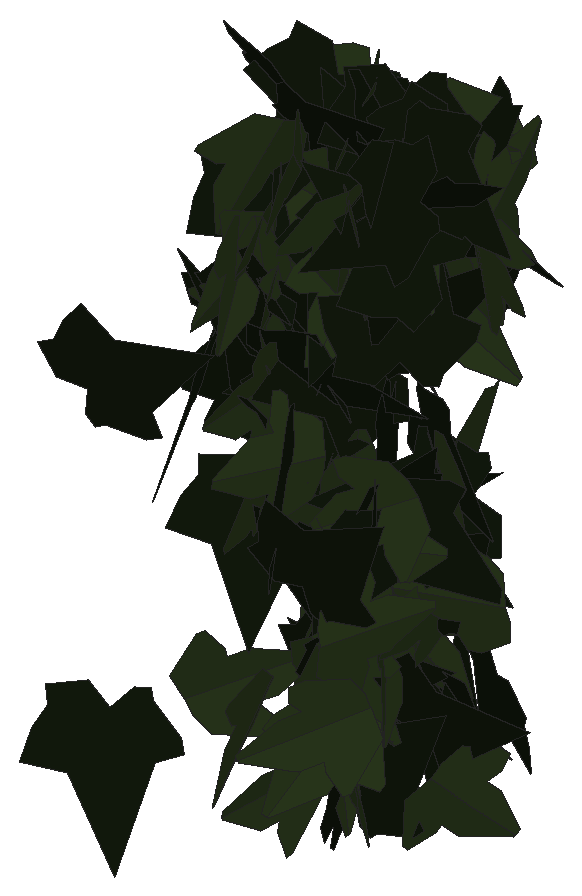
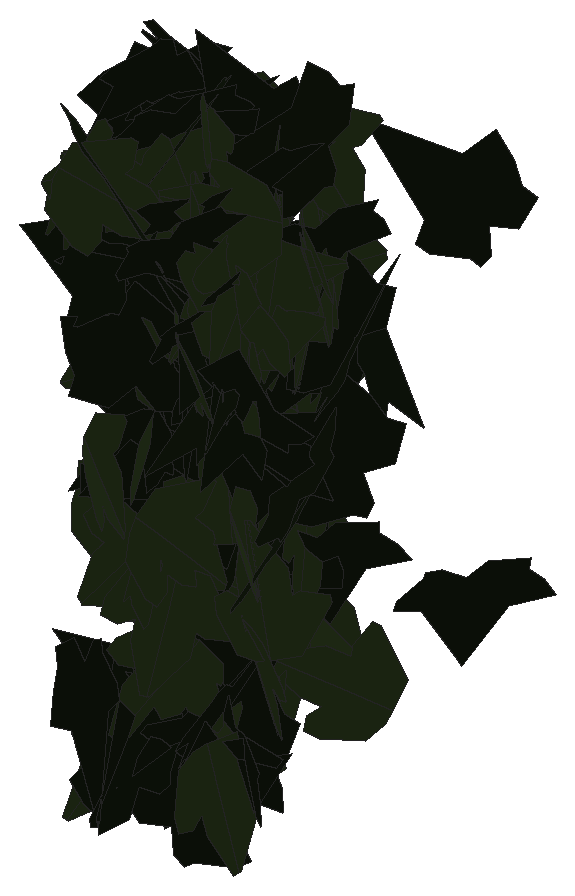
# SketchUp Ruby script. Lengths in inches.
U = 1.inch
M = Sketchup.active_model
def pt(a) = Geom::Point3d.new(a.map { |v| v * U })
def face(e, loops, mat)
  f = e.add_face(loops[0].map { |a| pt(a) })
  loops[1..].each { |l| e.add_face(l.map { |a| pt(a) }).erase! }
  f.material = f.back_material = mat if mat
  f
end
# faces: each face lists its corners as indices into pts; further lists are holes
def faces(e, pts, list, mat = nil) = list.each { |f| face(e, (f[0].is_a?(Array) ? f : [f]).map { |l| l.map { |i| pts[i] } }, mat) }
# xy, xz, yz: faces in a plane at the given z, y or x. An outline is a flat list of corners, or four numbers for a rectangle; further outlines are holes
def ring(l) = l.size == 4 ? [[l[0], l[1]], [l[2], l[1]], [l[2], l[3]], [l[0], l[3]]] : l.each_slice(2).to_a
def flat(e, list, mat, &to3) = list.each { |f| face(e, (f[0].is_a?(Array) ? f : [f]).map { |l| ring(l).map { |u, v| to3.(u, v) } }, mat) }
def xy(e, z, list, mat = nil) = flat(e, list, mat) { |x, y| [x, y, z] }
def xz(e, y, list, mat = nil) = flat(e, list, mat) { |x, z| [x, y, z] }
def yz(e, x, list, mat = nil) = flat(e, list, mat) { |y, z| [x, y, z] }
def lines(e, pts, list) = list.each { |a, b| e.add_line(pt(pts[a]), pt(pts[b])) }
# prism: a flat outline (further loops are holes) pulled along v
def prism(e, loops, v, mat = nil)
  f = face(e, loops, mat); d = Geom::Vector3d.new(v.map { |x| x * U })
  f.pushpull(f.normal.samedirection?(d) ? d.length : -d.length)
end
def box(e, o, s, mat = nil) = prism(e, [[o, [o[0] + s[0], o[1], o[2]], [o[0] + s[0], o[1] + s[1], o[2]], [o[0], o[1] + s[1], o[2]]]], [0, 0, s[2]], mat)
def at(x, y, z, deg = 0) = Geom::Transformation.translation(pt([x, y, z])) * Geom::Transformation.rotation(ORIGIN, Z_AXIS, deg.degrees)
def axes(o, x, y, z) = Geom::Transformation.new([*x, 0, *y, 0, *z, 0, *pt(o).to_a, 1])
def part(name) = M.definitions.add(name)
# library, detail: a bought-in or finely detailed component or shape, given as its bounding box
def library(name, o, s) = part(name).tap { |d| box(d.entities, o, s) }
def detail(e, o, s) = box(e.add_group.entities, o, s)
def put(e, d, t, mat = nil) = e.add_instance(d, t).tap { |i| i.material = mat if mat }
def group(e, t, mat = nil) = e.add_group.tap { |g| g.transformation = t; g.material = mat if mat }.entities
root = M.entities
M.materials.add("efeu1").color = [18, 25, 13]
M.materials.add("efeu2").color = [43, 57, 29]
c1 = part("ivyleaf_9")
p = [[1.54,2.16,1.25],[1.36,2.04,1.19],[-0.21,0.99,0.68],[-0.71,1.11,0.82],[-0.85,0.86,0.67],[-0.8,0.17,0.21],
  [-0.9,-0.01,0.1],[-0.67,-0.16,-0.02],[-0.08,-0.08,-0.05],[-0.03,-0.6,-0.4],[0.65,-0.88,-0.66],[0.83,-0.6,-0.49],
  [1.29,-0.42,-0.43],[1.8125,-0.07,-0.26],[1.21,0.44,0.15]]
faces(c1.entities,p,[[0,1,2,3,4,5,6,7,8,9,10,11,12,13,14]],"efeu1")
c2 = part("ivyleaf_10")
p = [[0,0.5,-0.03],[-0.0625,2.02,-0.43],[-0.19,2.01,-0.46],[-0.54,1.05,-0.29],[-0.52,0.625,-0.18],[-0.83,0.76,-0.28],
  [-1.16,0.64,-0.33],[-1.15,0.33,-0.24],[-0.77,-0.39,0.02],[-0.3,-0.51,0.16],[0.04,-0.48,0.23],[-0.02,2.01,-0.4375],
  [-0.06,2.01,-0.43],[0.04,-0.49,0.23],[0.67,-0.49,0.14],[1.38,0.36,-0.2],[1.375,0.51,-0.24],[0.81,0.65,-0.19],
  [0.62,0.59,-0.15],[0.6,1.09,-0.28],[0.5,1.23,-0.31]]
faces(c2.entities,p,[[0,1,2,3,4,5,6,7,8,9,10],[11,12,0,13,14,15,16,17,18,19,20]],"efeu2")
put(root,c1,axes([26.17,222.62,210.74],[0.16285,0.0009,0.47274],[0.47272,-0.00413,-0.16283],[0.00361,0.49998,-0.00219]))
put(root,c1,axes([26.61,221.9,211.7],[-0.299,0.15439,-0.36982],[0.31819,-0.18905,-0.33618],[-0.24363,-0.43638,0.0148]))
put(root,c1,axes([26.43,223.62,210.13],[0.05085,-0.39738,0.29918],[0.0403,-0.29645,-0.40061],[0.49577,0.06486,0.00187]))
put(root,c1,axes([26.73,222.37,211.34],[0.13991,-0.44603,0.17743],[-0.03757,0.17407,0.46721],[-0.47855,-0.14407,0.01519]))
put(root,c1,axes([26.56,222.69,209.89],[-0.24498,-0.39685,-0.18025],[0.10032,0.14988,-0.46634],[0.42417,-0.26465,0.00619]))
put(root,c1,axes([26.82,223.59,211.56],[-0.49386,0.06546,0.04259],[0.04104,-0.01442,0.4981],[0.06644,0.49549,0.00887]))
put(root,c1,axes([26.37,223.23,210.66],[0.11385,-0.33946,0.34901],[0.15332,-0.31519,-0.35658],[0.46209,0.18821,0.03232]))
put(root,c1,axes([26.55,220.52,208.52],[-0.17039,-0.42889,-0.19241],[0.07799,0.17603,-0.46144],[0.46356,-0.18727,0.00691]))
put(root,c2,axes([26.7,223.56,212.33],[-0.34285,-0.35172,-0.09353],[-0.05672,-0.07529,0.49103],[-0.3595,0.34731,0.01173]))
put(root,c2,axes([26.58,223.41,209.25],[-0.46251,-0.0941,0.16501],[0.168,0.00007,0.47093],[-0.08865,0.49107,0.03155]))
put(root,c2,axes([26.71,222.61,210.05],[0.03257,-0.4567,-0.20091],[0.0211,0.20242,-0.45671],[0.49849,0.02127,0.03246]))
put(root,c2,axes([26.47,222.11,208.01],[-0.14514,-0.17857,0.4439],[0.28518,0.34019,0.2301],[-0.3842,0.31997,0.0031]))
put(root,c1,axes([26.57,222.73,213.15],[-0.04749,-0.45954,-0.19123],[0.02534,0.18962,-0.46195],[0.49709,-0.05357,0.00528]))
put(root,c2,axes([26.81,223.9,207.91],[-0.12899,-0.47806,0.06942],[-0.02076,-0.0663,-0.49515],[0.48263,-0.13062,-0.00275]))
put(root,c2,axes([26.77,222.54,212.93],[0.19917,-0.45327,-0.06984],[-0.02871,0.06367,-0.4951],[0.45772,0.20122,-0.00066]))
put(root,c1,axes([26.37,222.87,214.1875],[0.37975,-0.23814,0.22154],[0.19105,-0.1123,-0.44821],[0.26323,0.42506,0.00571]))
put(root,c2,axes([26.72,223.39,213.05],[-0.28934,-0.35489,-0.20083],[0.13306,0.15061,-0.45784],[0.38546,-0.31839,0.00728]))
put(root,c2,axes([26.47,223.7,212.75],[0.3605,-0.05675,0.34178],[0.33953,-0.04033,-0.36482],[0.06897,0.49513,0.00946]))
put(root,c2,axes([26.99,222.3,211.92],[-0.01817,0.07692,0.49371],[-0.34311,0.35723,-0.06829],[-0.36324,-0.34128,0.03981]))
put(root,c2,axes([26.71,222.37,212.51],[0.01609,-0.11059,0.48735],[0.15839,-0.46134,-0.10992],[0.47398,0.15792,0.02019]))
put(root,c2,axes([26.77,223.36,209.04],[0.3873,-0.31618,0.00527],[0.00407,-0.00335,-0.49997],[0.31619,0.38733,-0.00003]))
put(root,c2,axes([26.58,222.82,213.16],[0.31779,-0.21999,0.3172],[0.26792,-0.1701,-0.38638],[0.27791,0.41554,0.00977]))
put(root,c2,axes([26.75,222.3,212.65],[0.02679,0.39052,-0.31109],[-0.0218,-0.31032,-0.39144],[-0.49881,0.03453,0.0004]))
put(root,c2,axes([27.07,223.27,212.69],[0.06772,0.08301,0.48839],[-0.30092,-0.38468,0.10711],[0.39353,-0.30844,-0.00215]))
put(root,c2,axes([26.91,222.375,213.78],[-0.12122,-0.43224,0.22017],[-0.05198,-0.21406,-0.44886],[0.48229,-0.13171,0.00696]))
put(root,c1,axes([27,223.26,211.625],[-0.12961,0.1107,-0.47005],[-0.35378,0.3095,0.17044],[0.3287,0.37677,-0.0019]))
put(root,c2,axes([26.88,222.42,212.07],[-0.41925,-0.26433,-0.06601],[-0.05587,-0.03515,0.49562],[-0.26666,0.42296,-0.00006]))
put(root,c1,axes([26.8,223.47,213.89],[-0.17872,-0.44691,0.13538],[-0.03161,-0.13304,-0.48094],[0.4659,-0.18047,0.0193]))
put(root,c1,axes([26.54,222.29,211.88],[0.17796,0.00183,0.46725],[0.46715,-0.01124,-0.17788],[0.00985,0.49987,-0.00571]))
put(root,c2,axes([26.89,223.4,210.18],[0.28334,-0.3892,0.13506],[0.07949,-0.1092,-0.48141],[0.40423,0.29428,-0.00001]))
put(root,c2,axes([26.61,223.58,213.65],[-0.05552,0.0027,-0.4969],[0.49367,-0.0567,-0.05547],[-0.05664,-0.49677,0.00362]))
put(root,c1,axes([26.75,223.78,211.89],[0.39734,-0.29675,-0.06375],[-0.04947,0.04031,-0.49591],[0.29946,0.40039,0.00268]))
put(root,c1,axes([26.71,222.87,212.0625],[0.30173,-0.39293,0.06761],[0.03483,-0.05849,-0.49534],[0.39718,0.30363,-0.00793]))
put(root,c2,axes([26.64,223.625,211.84],[-0.02809,0.00711,0.49916],[0.48941,-0.09821,0.02894],[0.09845,0.49021,-0.00144]))
put(root,c2,axes([26.98,222.85,212.16],[0.05224,-0.37634,0.32503],[0.10389,-0.31134,-0.37719],[0.48629,0.10695,0.04567]))
put(root,c1,axes([27.3125,223.84,207.17],[0.08373,-0.03379,0.49178],[-0.47208,0.13808,0.08987],[-0.14188,-0.47937,-0.00878]))
put(root,c1,axes([26.65,220.16,212.11],[0.03007,-0.01545,0.49886],[0.46411,-0.18295,-0.03365],[0.18357,0.46507,0.00334]))
put(root,c2,axes([27.14,222.42,213.66],[0.08173,-0.32712,-0.36921],[-0.0799,0.36052,-0.33711],[0.48676,0.1141,0.00666]))
put(root,c1,axes([27.08,222.48,209.71],[0.3855,0.18856,-0.25659],[-0.23497,-0.10345,-0.42905],[-0.21489,0.45138,0.00885]))
put(root,c1,axes([26.94,223.17,211.03],[-0.31527,-0.22643,-0.31517],[0.25376,0.18695,-0.38815],[0.29362,-0.4047,-0.00296]))
put(root,c1,axes([26.85,223.56,208.18],[-0.20134,-0.00646,-0.45763],[0.45766,0.00086,-0.20136],[0.00339,-0.49996,0.00556]))
put(root,c2,axes([27.08,222.23,211.36],[-0.03021,0.00692,-0.49904],[-0.09554,-0.49079,-0.00102],[-0.48986,0.09529,0.03097]))
put(root,c1,axes([26.91,223.55,208.57],[0.21902,-0.39966,-0.20567],[-0.10038,0.17952,-0.45574],[0.43813,0.24092,-0.0016]))
put(root,c1,axes([26.91,223.73,208.07],[-0.18921,-0.24159,-0.39476],[0.28116,0.27875,-0.30536],[0.36762,-0.33754,0.03036]))
put(root,c1,axes([27.39,222.8125,211.81],[-0.19338,0.14226,-0.4386],[-0.37892,0.22197,0.23906],[0.26273,0.42484,0.02196]))
put(root,c1,axes([27.05,223.83,212.6],[-0.08661,-0.47526,0.12893],[-0.01805,-0.12776,-0.48307],[0.49211,-0.08833,0.00497]))
put(root,c2,axes([27.08,223.61,212.87],[0.17,-0.46295,-0.08236],[0.02854,-0.07725,0.49317],[-0.46935,-0.17238,0.00016]))
put(root,c1,axes([27.18,224.05,213.43],[-0.20975,-0.45383,0.00682],[0.00304,-0.00892,-0.49991],[0.45387,-0.20967,0.0065]))
put(root,c2,axes([27.12,223.93,212.1875],[0.36105,-0.30275,0.16728],[0.13199,-0.10293,-0.47115],[0.31972,0.38438,0.00559]))
put(root,c1,axes([26.84,223.33,207.8],[0.12129,-0.04112,0.48332],[0.44543,-0.1878,-0.12776],[0.19205,0.46156,-0.00892]))
put(root,c2,axes([26.99,223.54,211.42],[-0.15248,0.09097,0.46741],[0.40194,-0.23857,0.17756],[0.25533,0.42989,-0.00037]))
put(root,c1,axes([27.39,223.19,212.24],[0.00918,0.37993,0.32491],[-0.00873,0.32504,-0.37983],[-0.49984,0.0013,0.0126]))
put(root,c2,axes([27.26,223.11,212.69],[-0.05645,0.32084,0.37931],[-0.05751,0.37497,-0.32572],[-0.49346,-0.0804,-0.00543]))
put(root,c2,axes([27.38,222.23,210.68],[-0.07152,0.10628,0.48331],[0.0082,-0.48801,0.10853],[0.49479,0.02345,0.06806]))
put(root,c2,axes([27.32,221.69,208.41],[0.16962,-0.34433,0.32041],[0.12132,-0.29705,-0.38346],[0.45443,0.20783,-0.01722]))
put(root,c2,axes([27.17,223.5,207.66],[-0.25968,0.05327,0.42394],[0.36467,-0.23091,0.25239],[0.22268,0.44027,0.08107]))
put(root,c2,axes([27.5,223.08,214.14],[0.15363,-0.4324,-0.19857],[-0.06775,0.18666,-0.45888],[0.47097,0.1679,-0.00124]))
put(root,c1,axes([27.59,223.03,211.4],[-0.04342,-0.28725,-0.40694],[-0.00307,-0.40833,0.28855],[-0.4981,0.02756,0.0337]))
put(root,c2,axes([27.04,222.81,213.04],[0.06665,0.02183,0.49506],[0.47473,0.1404,-0.0701],[-0.14208,0.47939,-0.00201]))
put(root,c1,axes([27.13,222.74,213.76],[0.44945,0.0194,-0.21822],[0.21512,0.05529,0.44796],[0.04151,-0.49656,0.04135]))
put(root,c1,axes([27.32,222.09,210.96],[-0.17708,-0.00608,-0.46755],[0.4513,-0.13304,-0.16919],[-0.12235,-0.48194,0.05261]))
put(root,c1,axes([27.09,222.31,211.55],[0.36588,-0.0643,0.33466],[0.33245,-0.04054,-0.37126],[0.07488,0.49419,0.01309]))
put(root,c1,axes([27.22,223.35,213.31],[0.07971,-0.25879,-0.42032],[0.16006,0.41631,-0.22597],[0.46693,-0.09853,0.14921]))
put(root,c2,axes([27.5,222.84,209.9],[-0.29594,-0.40274,-0.01499],[-0.00129,-0.01765,0.49969],[-0.40301,0.29579,0.00941]))
put(root,c1,axes([27.46,223.01,212.57],[-0.1235,-0.46146,0.14767],[-0.02387,-0.14641,-0.47749],[0.48392,-0.12499,0.01413]))
put(root,c2,axes([27.49,222.67,207.79],[-0.02474,0.49661,-0.05256],[-0.00154,-0.0527,-0.49721],[-0.49939,-0.02444,0.00414]))
put(root,c1,axes([27.62,222.47,206.99],[0.0529,-0.09327,0.48837],[0.1044,0.48226,0.08079],[-0.48611,0.09343,0.0705]))
put(root,c1,axes([27.6,222.71,208.75],[0.22704,0.44385,0.03807],[0.01667,0.03423,-0.49855],[-0.44517,0.22765,0.00075]))
put(root,c2,axes([27.73,223.6,209.96],[-0.02025,-0.35618,0.35032],[-0.02928,-0.34916,-0.3567],[0.49873,-0.03497,-0.00672]))
put(root,c2,axes([27.51,222.54,208.58],[-0.42571,-0.00681,-0.26215],[0.26207,0.00693,-0.42576],[0.00943,-0.49991,-0.00233]))
put(root,c1,axes([28.08,223.63,212.52],[-0.34273,0.1301,0.34002],[-0.32111,0.11202,-0.36653],[-0.17154,-0.4696,0.00677]))
put(root,c2,axes([27.73,223.41,209.25],[-0.46418,-0.17554,-0.06101],[0.05644,0.02321,-0.49626],[0.17706,-0.4676,-0.00173]))
put(root,c2,axes([27.76,221.8,207.72],[-0.00342,0.01262,-0.49983],[-0.15199,-0.47621,-0.01099],[-0.47633,0.15186,0.0071]))
put(root,c2,axes([27.59,223.45,208.6],[-0.41899,-0.08519,-0.25921],[0.25243,0.05927,-0.42751],[0.10357,-0.48911,-0.00666]))
put(root,c1,axes([27.74,223.89,211.7],[0.34593,0.11689,0.34157],[-0.32158,-0.11523,0.36511],[0.16408,-0.47229,-0.00454]))
put(root,c2,axes([27.52,223.26,212.31],[-0.27243,0.0022,0.41926],[0.41918,0.01135,0.27232],[-0.00832,0.49987,-0.00803]))
put(root,c2,axes([27.89,222.47,212.73],[0.38533,0.25472,-0.1914],[-0.16178,-0.10234,-0.4619],[-0.27449,0.4179,0.00354]))
put(root,c1,axes([28.17,222.58,213.44],[-0.47342,-0.12768,-0.09784],[-0.09464,-0.0248,0.49033],[-0.13006,0.48279,-0.00069]))
put(root,c2,axes([27.89,222.41,207.24],[-0.41132,0.25837,0.11859],[0.09753,-0.06767,0.4857],[0.26703,0.42269,0.00527]))
put(root,c1,axes([27.62,222.79,207.1],[-0.14312,0.06557,0.47457],[0.39325,-0.26681,0.15546],[0.27363,0.41775,0.02481]))
put(root,c1,axes([27.64,223.25,214.06],[0.22911,-0.44398,0.01987],[0.01278,-0.01577,-0.49959],[0.44424,0.22942,0.00412]))
put(root,c1,axes([27.5625,222.64,209.47],[0.31401,-0.12379,-0.36888],[0.35745,-0.09548,0.33632],[-0.15371,-0.47493,0.02853]))
put(root,c2,axes([27.875,223.23,213.68],[0.28411,0.39303,-0.12171],[-0.08054,-0.09192,-0.48483],[-0.40348,0.29509,0.01108]))
put(root,c1,axes([27.8,223.23,214.15],[-0.11782,-0.46469,-0.14205],[0.03113,0.13865,-0.47938],[0.48492,-0.1218,-0.00374]))
put(root,c1,axes([27.64,224,207.56],[0.46096,-0.1147,-0.15607],[0.1563,-0.01764,0.47461],[-0.11438,-0.48635,0.01959]))
put(root,c2,axes([28.3,223.99,213.59],[-0.16842,-0.11853,0.45562],[-0.34684,-0.29596,-0.20521],[0.31834,-0.38517,0.01747]))
put(root,c2,axes([27.87,222.95,208.73],[-0.09098,0.37961,-0.31245],[0.08435,-0.30099,-0.39025],[-0.48436,-0.12371,-0.00927]))
put(root,c2,axes([28.06,222.02,213.625],[-0.11435,-0.48505,-0.04058],[0.00527,0.04045,-0.49833],[0.48672,-0.11439,-0.00414]))
put(root,c1,axes([28.14,223.57,207.14],[-0.06621,-0.28754,0.40365],[0.13509,0.38135,0.29381],[-0.47683,0.14796,0.02718]))
put(root,c2,axes([27.95,222.23,213.52],[-0.2488,0.37033,-0.22573],[0.11555,-0.19423,-0.44601],[-0.41803,-0.2741,0.01106]))
put(root,c2,axes([27.75,223.59,213.34],[-0.16853,-0.08475,0.46305],[0.42561,0.18272,0.18834],[-0.20114,0.45764,0.01055]))
put(root,c1,axes([27.9,222.89,211.125],[-0.08364,0.0526,-0.49014],[0.43778,-0.22061,-0.09838],[-0.22661,-0.4456,-0.00915]))
put(root,c2,axes([27.81,223.64,211.81],[0.21812,0.11261,0.4356],[0.39599,0.18175,-0.24527],[-0.21358,0.45198,-0.0099]))
put(root,c2,axes([28.48,222.22,210.625],[0.27616,-0.00071,-0.41682],[-0.41165,0.07799,-0.27287],[0.0654,0.49388,0.04249]))
put(root,c1,axes([28.54,223.48,213.63],[-0.27868,0.3462,0.22908],[-0.13841,0.18264,-0.44439],[-0.39138,-0.3111,-0.00596]))
put(root,c2,axes([28.17,223.9375,210.74],[0.19972,-0.42067,0.18207],[0.09667,-0.15547,-0.46528],[0.44807,0.22105,0.01923]))
put(root,c2,axes([28.05,223.54,209.66],[-0.37779,0.16182,-0.28477],[0.26304,-0.10914,-0.41098],[-0.19517,-0.46033,-0.00266]))
put(root,c1,axes([28.56,223.17,210.3125],[-0.13626,-0.21746,-0.42912],[-0.19751,-0.38139,0.25599],[-0.43866,0.23927,0.01804]))
put(root,c2,axes([28.48,221.51,208.7],[0.12869,0.11251,-0.46987],[-0.37614,-0.28187,-0.17051],[-0.30325,0.39736,0.01209]))
put(root,c1,axes([28.12,222.4375,210.26],[0.18933,0.23912,0.3962],[0.23952,0.31564,-0.30496],[-0.39596,0.30527,0.00498]))
put(root,c2,axes([28.35,221.54,208.57],[0.304,0.26365,-0.29676],[-0.22117,-0.19791,-0.40239],[-0.32965,0.37592,-0.00371]))
put(root,c1,axes([28.26,223.26,213.84],[-0.21369,-0.42935,0.1414],[-0.05618,-0.12997,-0.47953],[0.44853,-0.22083,0.0073]))
put(root,c2,axes([28.25,223.2,209.16],[-0.00413,-0.04106,0.49829],[0.16037,-0.47209,-0.03757],[0.47356,0.15952,0.01707]))
put(root,c1,axes([27.94,223.15,207.75],[0.1279,-0.05738,0.47995],[0.42079,-0.23108,-0.13976],[0.23786,0.43967,-0.01082]))
put(root,c1,axes([27.95,223.875,212.79],[0.25917,-0.25474,0.34343],[0.29152,-0.18852,-0.35983],[0.31281,0.38674,0.05081]))
put(root,c1,axes([28.0625,221.47,209.99],[-0.11324,-0.06043,0.48325],[0.41409,-0.27308,0.06289],[0.25633,0.41446,0.11189]))
put(root,c2,axes([28.25,222.36,213.375],[0.12269,0.42821,0.22712],[0.06557,0.21747,-0.44543],[-0.48026,0.13908,-0.00279]))
put(root,c2,axes([28,222.33,210.01],[0.0892,-0.0706,-0.48689],[0.47788,-0.10516,0.1028],[-0.11692,-0.48369,0.04872]))
put(root,c1,axes([28.57,223.61,208.24],[0.23204,0.02557,-0.44216],[-0.4413,-0.02893,-0.23327],[-0.03751,0.49851,0.00914]))
put(root,c2,axes([28.27,221.72,209.4],[0.0017,-0.02643,-0.4993],[0.24581,0.43484,-0.02218],[0.4354,-0.24539,0.01447]))
put(root,c1,axes([28.44,222.37,212.09],[-0.38914,-0.10648,0.29535],[0.28576,0.07469,0.40344],[-0.13003,0.48279,0.00273]))
put(root,c1,axes([28.16,223.09,209.21],[-0.14507,-0.03097,0.47749],[0.37198,-0.32114,0.09218],[0.30097,0.38198,0.11622]))
put(root,c2,axes([28.43,223.34,212.9],[-0.48115,-0.11119,-0.07828],[0.07591,0.01919,-0.49383],[0.11283,-0.4871,-0.00159]))
put(root,c1,axes([28.3125,222.54,212.14],[0.07572,0.10053,0.4839],[0.33876,0.34591,-0.12487],[-0.35988,0.34676,-0.01573]))
put(root,c1,axes([28.77,222.34,213.18],[-0.29235,-0.38635,-0.12355],[-0.07372,-0.09915,0.48449],[-0.39887,0.3015,0.00101]))
put(root,c1,axes([28.12,223.14,210.91],[0.08292,-0.05119,-0.49041],[0.49116,0.05236,0.07759],[0.04341,-0.49461,0.05896]))
put(root,c2,axes([28.34,223.1,210.66],[-0.29011,0.30654,-0.26809],[0.17814,-0.20047,-0.42199],[-0.36621,-0.34036,0.00711]))
put(root,c2,axes([28.66,223.31,212.81],[-0.44178,0.19036,0.13635],[-0.12656,0.05084,-0.48104],[-0.19701,-0.45954,0.00327]))
put(root,c2,axes([28.48,222.99,207.36],[-0.2077,-0.30243,-0.3397],[0.2007,0.27418,-0.3668],[0.40814,-0.28873,0.0075]))
put(root,c1,axes([28.5625,222.3,213.66],[0.26143,0.42218,0.0585],[0.03126,0.04945,-0.49657],[-0.42506,0.26329,-0.00054]))
put(root,c1,axes([28.89,222.02,213.97],[-0.47488,0.13158,0.08472],[-0.08029,0.02749,-0.49274],[-0.13432,-0.48159,-0.00498]))
put(root,c1,axes([28.35,222.27,210.44],[0.00554,-0.09489,-0.49088],[0.17233,0.46119,-0.08721],[0.46933,-0.16822,0.03781]))
put(root,c1,axes([28.44,222.48,214.18],[0.1294,-0.28194,-0.39213],[-0.02199,0.4021,-0.29637],[0.48246,0.09394,0.09166]))
put(root,c2,axes([29.02,222.88,209.51],[-0.06891,-0.00994,0.49513],[-0.47478,-0.14084,-0.06891],[0.14083,-0.47965,0.00997]))
put(root,c2,axes([28.7,223.375,213.3],[0.01824,0.18023,-0.46603],[0.01498,0.46593,0.18078],[0.49944,-0.02056,0.01159]))
